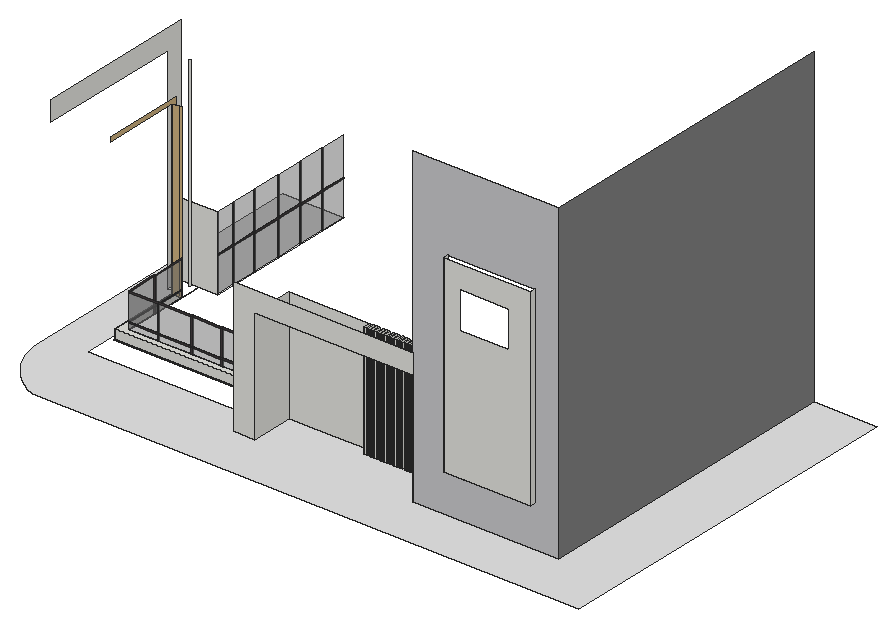
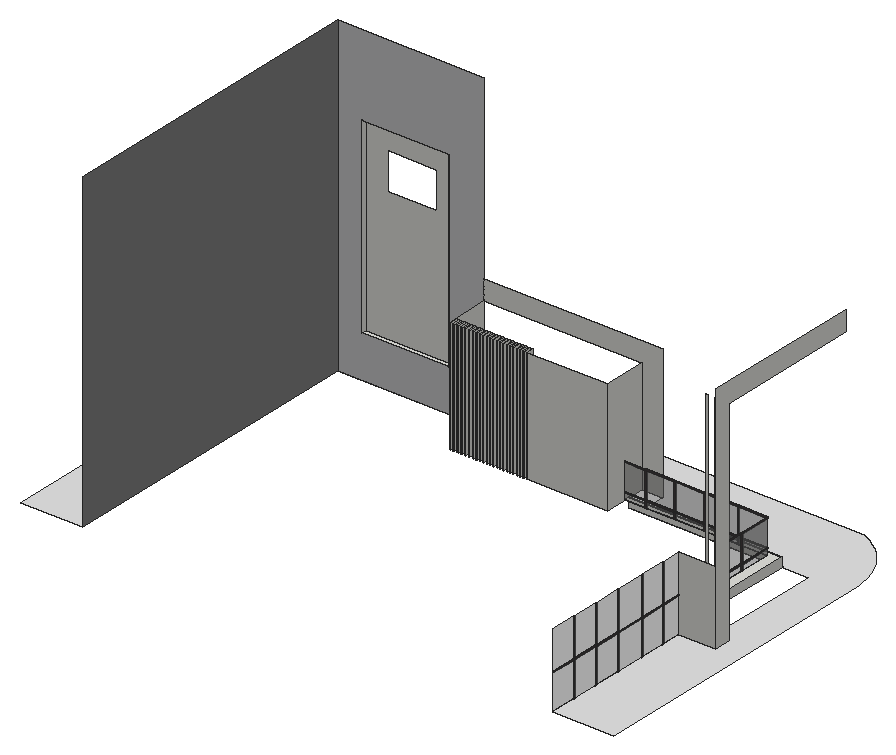
# SketchUp Ruby script. Lengths in inches.
U = 1.inch
M = Sketchup.active_model
def pt(a) = Geom::Point3d.new(a.map { |v| v * U })
def face(e, loops, mat)
  f = e.add_face(loops[0].map { |a| pt(a) })
  loops[1..].each { |l| e.add_face(l.map { |a| pt(a) }).erase! }
  f.material = f.back_material = mat if mat
  f
end
# faces: each face lists its corners as indices into pts; further lists are holes
def faces(e, pts, list, mat = nil) = list.each { |f| face(e, (f[0].is_a?(Array) ? f : [f]).map { |l| l.map { |i| pts[i] } }, mat) }
# xy, xz, yz: faces in a plane at the given z, y or x. An outline is a flat list of corners, or four numbers for a rectangle; further outlines are holes
def ring(l) = l.size == 4 ? [[l[0], l[1]], [l[2], l[1]], [l[2], l[3]], [l[0], l[3]]] : l.each_slice(2).to_a
def flat(e, list, mat, &to3) = list.each { |f| face(e, (f[0].is_a?(Array) ? f : [f]).map { |l| ring(l).map { |u, v| to3.(u, v) } }, mat) }
def xy(e, z, list, mat = nil) = flat(e, list, mat) { |x, y| [x, y, z] }
def xz(e, y, list, mat = nil) = flat(e, list, mat) { |x, z| [x, y, z] }
def yz(e, x, list, mat = nil) = flat(e, list, mat) { |y, z| [x, y, z] }
def lines(e, pts, list) = list.each { |a, b| e.add_line(pt(pts[a]), pt(pts[b])) }
# prism: a flat outline (further loops are holes) pulled along v
def prism(e, loops, v, mat = nil)
  f = face(e, loops, mat); d = Geom::Vector3d.new(v.map { |x| x * U })
  f.pushpull(f.normal.samedirection?(d) ? d.length : -d.length)
end
def box(e, o, s, mat = nil) = prism(e, [[o, [o[0] + s[0], o[1], o[2]], [o[0] + s[0], o[1] + s[1], o[2]], [o[0], o[1] + s[1], o[2]]]], [0, 0, s[2]], mat)
def at(x, y, z, deg = 0) = Geom::Transformation.translation(pt([x, y, z])) * Geom::Transformation.rotation(ORIGIN, Z_AXIS, deg.degrees)
def axes(o, x, y, z) = Geom::Transformation.new([*x, 0, *y, 0, *z, 0, *pt(o).to_a, 1])
def part(name) = M.definitions.add(name)
# library, detail: a bought-in or finely detailed component or shape, given as its bounding box
def library(name, o, s) = part(name).tap { |d| box(d.entities, o, s) }
def detail(e, o, s) = box(e.add_group.entities, o, s)
def put(e, d, t, mat = nil) = e.add_instance(d, t).tap { |i| i.material = mat if mat }
def group(e, t, mat = nil) = e.add_group.tap { |g| g.transformation = t; g.material = mat if mat }.entities
root = M.entities
M.materials.add("[0133_Gray]").color = [128, 128, 128]
M.materials.add("[Asphalt New]").color = [67, 60, 62]
M.materials.add("[Polished Concrete New]").color = [200, 200, 203]
M.materials.add("[Polished Concrete Old]").color = [229, 229, 229]
M.materials.add("[Translucent Glass Gray]").color = [128, 128, 128]
M.materials["[Translucent Glass Gray]"].alpha = 0.5
M.materials.add("[Wood Floor Light]").color = [204, 176, 127]
xy(root,1.5625,[[560.04,113.86,967.75,113.86,967.75,390.8,921.28,390.8,921.28,152.69,812.47,152.69,812.47,184.77,811.54,184.77,811.54,179.27,809.84,179.27,809.84,184.77,808.66,184.77,808.66,179.27,806.97,179.27,806.97,184.77,805.79,184.77,805.79,179.27,804.09,179.27,804.09,184.77,802.91,184.77,802.91,179.27,801.22,179.27,801.22,184.77,800.04,184.77,800.04,179.27,798.34,179.27,798.34,184.77,797.16,184.77,797.16,179.27,795.47,179.27,795.47,184.77,794.29,184.77,794.29,179.27,792.59,179.27,792.59,184.77,791.79,184.77,791.79,179.27,790.09,179.27,790.09,184.77,789.29,184.77,789.29,179.27,787.59,179.27,787.59,184.77,786.79,184.77,786.79,179.27,785.09,179.27,785.09,184.77,784.29,184.77,784.29,179.27,782.59,179.27,782.59,184.77,781.79,184.77,781.79,179.27,780.09,179.27,780.09,184.77,779.29,184.77,779.29,179.27,777.59,179.27,777.59,184.77,776.79,184.77,776.79,179.27,775.09,179.27,775.09,184.77,774.29,184.77,774.29,179.27,772.59,179.27,772.59,184.77,771.79,184.77,771.79,179.27,770.09,179.27,770.09,184.77,769.29,184.77,769.29,179.27,767.59,179.27,767.59,184.77,766.79,184.77,766.79,179.27,765.09,179.27,765.09,184.77,764.29,184.77,764.29,179.27,762.59,179.27,762.59,184.77,761.79,184.77,761.79,179.27,760.09,179.27,760.09,184.77,759.29,184.77,759.29,179.27,757.59,179.27,757.59,184.77,756.79,184.77,756.79,179.27,755.09,179.27,755.09,184.77,694.73,184.77,694.73,152.69,679.09,152.69,679.09,173.38,553.86,173.38,553.86,261.08,542.91,261.08,542.91,273.58,570.41,273.58,570.41,390.8,525.25,390.8,525.25,162.48,525.49,159.18,526.54,153.3125,528.21,147.58,530.47,142.06,533.3,136.8,536.66,131.87,540.53,127.32,544.85,123.2,549.57,119.56,554.66,116.43]],"[Polished Concrete Old]")
xy(root,9.25,[[565.04,183.7,679.09,184.6],[565.04,237.58,565.41,237.58,565.41,241.02,565.16,241.02,565.16,261.08,565.04,261.08]])
xy(root,16.125,[[565.04,184.6,679.09,184.6,679.09,188.52,572.41,188.52,572.41,237.58,565.04,237.58]])
xy(root,32.7,[[839.12,148.44,903.81,152.69]])
xz(root,148.44,[[[839.12,32.7,903.81,175.33],[850.82,130.92,887.85,158.83]]])
xz(root,152.69,[[679.09,1.5625,694.73,1.5625,694.73,86.125,812.47,86.125,812.47,101.125,679.09,101.125]])
xz(root,152.69,[[[812.47,1.5625,921.28,235.625],[839.12,32.7,903.81,175.33]]],"[Polished Concrete New]")
xz(root,179.27,[[755.09,1.5625,756.79,86.125],[757.59,1.5625,759.29,86.125],[760.09,1.5625,761.79,86.125],[762.59,1.5625,764.29,86.125],[765.09,1.5625,766.79,86.125],
  [767.59,1.5625,769.29,86.125],[770.09,1.5625,771.79,86.125],[772.59,1.5625,774.29,86.125],[775.09,1.5625,776.79,86.125],[777.59,1.5625,779.29,86.125],
  [780.09,1.5625,781.79,86.125],[782.59,1.5625,784.29,86.125],[785.09,1.5625,786.79,86.125],[787.59,1.5625,789.29,86.125],[790.09,1.5625,791.79,86.125],
  [792.59,1.5625,794.29,86.125],[795.47,1.5625,797.16,86.125],[798.34,1.5625,800.04,86.125],[801.22,1.5625,802.91,86.125],[804.09,1.5625,805.79,86.125],
  [806.97,1.5625,808.66,86.125],[809.84,1.5625,811.54,86.125]])
xz(root,184.6,[[565.04,9.25,679.09,16.125]])
xz(root,184.77,[[694.73,1.5625,755.09,86.125],[756.79,1.5625,757.59,86.125],[759.29,1.5625,760.09,86.125],[761.79,1.5625,762.59,86.125],[764.29,1.5625,765.09,86.125],
  [766.79,1.5625,767.59,86.125],[769.29,1.5625,770.09,86.125],[771.79,1.5625,772.59,86.125],[774.29,1.5625,775.09,86.125],[776.79,1.5625,777.59,86.125],
  [779.29,1.5625,780.09,86.125],[781.79,1.5625,782.59,86.125],[784.29,1.5625,785.09,86.125],[786.79,1.5625,787.59,86.125],[789.29,1.5625,790.09,86.125],
  [791.79,1.5625,792.59,86.125],[794.29,1.5625,795.47,86.125],[797.16,1.5625,798.34,86.125],[800.04,1.5625,801.22,86.125],[802.91,1.5625,804.09,86.125],
  [805.79,1.5625,806.97,86.125],[808.66,1.5625,809.84,86.125],[811.54,1.5625,812.47,86.125]])
xz(root,188.52,[[593.95,16.125,594.71,20.57],[618.47,16.125,619.6,20.57],[641.13,16.125,642.0625,20.57],[662.45,16.125,663.59,20.57],[572.41,20.57,593.95,21.6],
  [593.95,20.57,594.71,21.6],[594.71,20.57,618.47,21.6],[618.47,20.57,619.6,21.6],[619.6,20.57,641.13,21.6],[641.13,20.57,642.0625,21.6],
  [642.0625,20.57,662.45,21.6],[662.45,20.57,663.59,21.6],[663.59,20.57,679.09,21.6],[593.95,21.6,594.71,41.14],[618.47,21.6,619.6,41.14],
  [641.13,21.6,642.0625,41.14],[662.45,21.6,663.59,41.14],[572.41,41.14,593.95,42.44],[593.95,41.14,594.71,42.44],[594.71,41.14,618.47,42.44],
  [618.47,41.14,619.6,42.44],[619.6,41.14,641.13,42.44],[641.13,41.14,642.0625,42.44],[642.0625,41.14,662.45,42.44],[662.45,41.14,663.59,42.44],
  [663.59,41.14,679.09,42.44]],"[Asphalt New]")
xz(root,188.52,[[572.41,16.125,593.95,20.57],[594.71,16.125,618.47,20.57],[619.6,16.125,641.13,20.57],[642.0625,16.125,662.45,20.57],[663.59,16.125,679.09,20.57],
  [572.41,21.6,593.95,41.14],[594.71,21.6,618.47,41.14],[619.6,21.6,641.13,41.14],[642.0625,21.6,662.45,41.14],[663.59,21.6,679.09,41.14]],"[Translucent Glass Gray]")
xz(root,237.58,[[565.04,9.25,565.41,16.125]])
xz(root,237.58,[[565.41,16.125,570.41,143.35],[570.41,16.125,572.41,143.35]],"[Wood Floor Light]")
xz(root,261.08,[[559.28,9.25,560.36,160.15]])
xz(root,273.58,[[542.91,1.5625,570.41,56.77]])
yz(root,542.91,[[261.08,1.5625,261.08,160.15,152.69,160.15,152.69,175.35,273.58,175.35,273.58,1.5625]])
yz(root,565.04,[[184.6,9.25,237.58,16.125]])
yz(root,565.41,[[237.58,9.25,237.58,143.35,179.89,143.35,179.89,146.5,241.02,146.5,241.02,9.25]],"[Wood Floor Light]")
yz(root,570.41,[[288.11,1.5625,288.9,27.2],[307.55,1.5625,308.36,27.2],[329.67,1.5625,330.36,27.2],[350.49,1.5625,350.93,27.2],[370.6875,1.5625,371.49,27.2],
  [273.58,27.2,288.11,28.38],[288.11,27.2,288.9,28.38],[288.9,27.2,307.55,28.38],[307.55,27.2,308.36,28.38],[308.36,27.2,329.67,28.38],
  [329.67,27.2,330.36,28.38],[330.36,27.2,350.49,28.38],[350.49,27.2,350.93,28.38],[350.93,27.2,370.6875,28.38],[370.6875,27.2,371.49,28.38],
  [371.49,27.2,390.8,28.38],[288.11,28.38,288.9,56.77],[307.55,28.38,308.36,56.77],[329.67,28.38,330.36,56.77],[350.49,28.38,350.93,56.77],
  [370.6875,28.38,371.49,56.77]],"[Asphalt New]")
yz(root,570.41,[[273.58,1.5625,288.11,27.2],[288.9,1.5625,307.55,27.2],[308.36,1.5625,329.67,27.2],[330.36,1.5625,350.49,27.2],[350.93,1.5625,370.6875,27.2],
  [371.49,1.5625,390.8,27.2],[273.58,28.38,288.11,56.77],[288.9,28.38,307.55,56.77],[308.36,28.38,329.67,56.77],[330.36,28.38,350.49,56.77],
  [350.93,28.38,370.6875,56.77],[371.49,28.38,390.8,56.77]],"[Translucent Glass Gray]")
yz(root,572.41,[[211.54,16.125,213.05,20.57],[188.52,20.57,210.03,21.6],[210.03,20.57,211.54,21.6],[211.54,20.57,213.05,21.6],[213.05,20.57,237.58,21.6],
  [211.54,21.6,213.05,41.14],[188.52,41.14,210.03,42.44],[210.03,41.14,211.54,42.44],[211.54,41.14,213.05,42.44],[213.05,41.14,237.58,42.44]],"[Asphalt New]")
yz(root,572.41,[[188.52,16.125,211.54,20.57],[213.05,16.125,237.58,20.57],[188.52,21.6,211.54,41.14],[213.05,21.6,237.58,41.14]],"[Translucent Glass Gray]")
yz(root,694.73,[[152.69,1.5625,184.77,86.125]])
yz(root,755.09,[[179.27,1.5625,184.77,86.125]])
yz(root,756.79,[[179.27,1.5625,184.77,86.125]])
yz(root,757.59,[[179.27,1.5625,184.77,86.125]])
yz(root,759.29,[[179.27,1.5625,184.77,86.125]])
yz(root,760.09,[[179.27,1.5625,184.77,86.125]])
yz(root,761.79,[[179.27,1.5625,184.77,86.125]])
yz(root,762.59,[[179.27,1.5625,184.77,86.125]])
yz(root,764.29,[[179.27,1.5625,184.77,86.125]])
yz(root,765.09,[[179.27,1.5625,184.77,86.125]])
yz(root,766.79,[[179.27,1.5625,184.77,86.125]])
yz(root,767.59,[[179.27,1.5625,184.77,86.125]])
yz(root,769.29,[[179.27,1.5625,184.77,86.125]])
yz(root,770.09,[[179.27,1.5625,184.77,86.125]])
yz(root,771.79,[[179.27,1.5625,184.77,86.125]])
yz(root,772.59,[[179.27,1.5625,184.77,86.125]])
yz(root,774.29,[[179.27,1.5625,184.77,86.125]])
yz(root,775.09,[[179.27,1.5625,184.77,86.125]])
yz(root,776.79,[[179.27,1.5625,184.77,86.125]])
yz(root,777.59,[[179.27,1.5625,184.77,86.125]])
yz(root,779.29,[[179.27,1.5625,184.77,86.125]])
yz(root,780.09,[[179.27,1.5625,184.77,86.125]])
yz(root,781.79,[[179.27,1.5625,184.77,86.125]])
yz(root,782.59,[[179.27,1.5625,184.77,86.125]])
yz(root,784.29,[[179.27,1.5625,184.77,86.125]])
yz(root,785.09,[[179.27,1.5625,184.77,86.125]])
yz(root,786.79,[[179.27,1.5625,184.77,86.125]])
yz(root,787.59,[[179.27,1.5625,184.77,86.125]])
yz(root,789.29,[[179.27,1.5625,184.77,86.125]])
yz(root,790.09,[[179.27,1.5625,184.77,86.125]])
yz(root,791.79,[[179.27,1.5625,184.77,86.125]])
yz(root,792.59,[[179.27,1.5625,184.77,86.125]])
yz(root,794.29,[[179.27,1.5625,184.77,86.125]])
yz(root,795.47,[[179.27,1.5625,184.77,86.125]])
yz(root,797.16,[[179.27,1.5625,184.77,86.125]])
yz(root,798.34,[[179.27,1.5625,184.77,86.125]])
yz(root,800.04,[[179.27,1.5625,184.77,86.125]])
yz(root,801.22,[[179.27,1.5625,184.77,86.125]])
yz(root,802.91,[[179.27,1.5625,184.77,86.125]])
yz(root,804.09,[[179.27,1.5625,184.77,86.125]])
yz(root,805.79,[[179.27,1.5625,184.77,86.125]])
yz(root,806.97,[[179.27,1.5625,184.77,86.125]])
yz(root,808.66,[[179.27,1.5625,184.77,86.125]])
yz(root,809.84,[[179.27,1.5625,184.77,86.125]])
yz(root,811.54,[[179.27,1.5625,184.77,86.125]])
yz(root,812.47,[[152.69,1.5625,184.77,86.125]])
yz(root,839.12,[[148.44,32.7,152.69,175.33]])
yz(root,903.81,[[148.44,32.7,152.69,175.33]])
yz(root,921.28,[[152.69,1.5625,390.8,235.625]],"[0133_Gray]")
